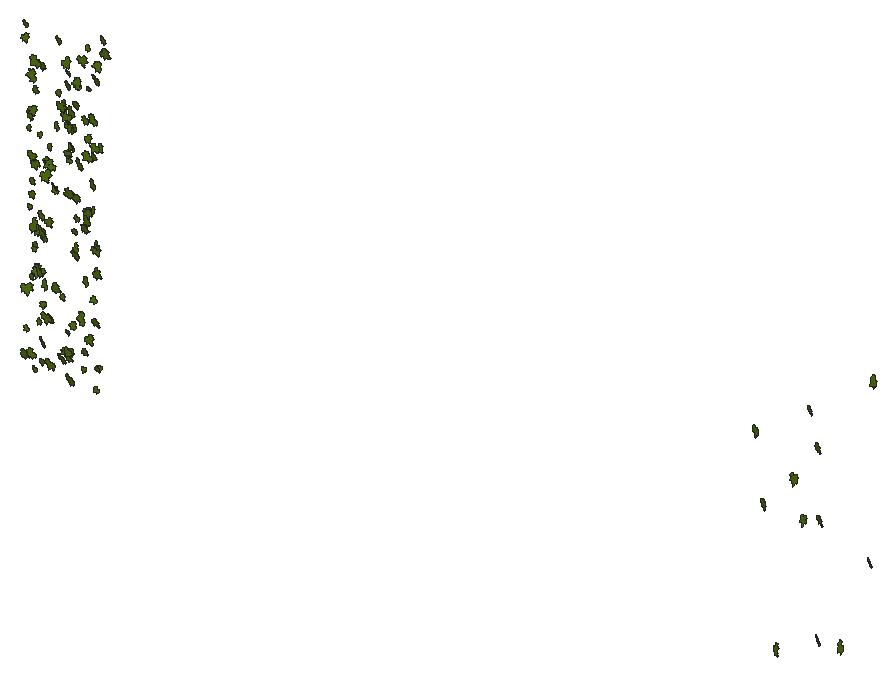
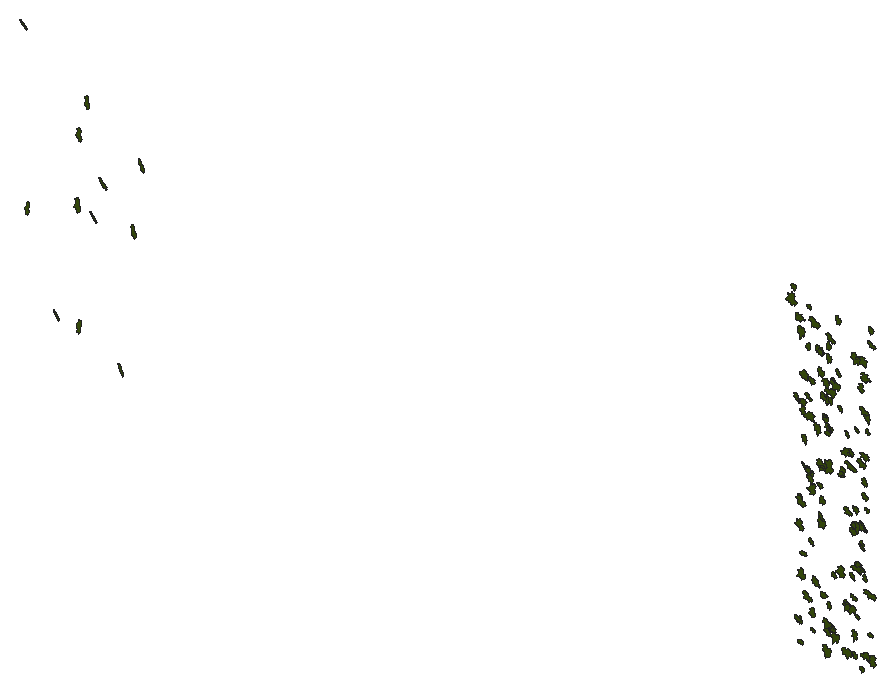
# SketchUp Ruby script. Lengths in inches.
U = 1.inch
M = Sketchup.active_model
def pt(a) = Geom::Point3d.new(a.map { |v| v * U })
def face(e, loops, mat)
  f = e.add_face(loops[0].map { |a| pt(a) })
  loops[1..].each { |l| e.add_face(l.map { |a| pt(a) }).erase! }
  f.material = f.back_material = mat if mat
  f
end
# faces: each face lists its corners as indices into pts; further lists are holes
def faces(e, pts, list, mat = nil) = list.each { |f| face(e, (f[0].is_a?(Array) ? f : [f]).map { |l| l.map { |i| pts[i] } }, mat) }
# xy, xz, yz: faces in a plane at the given z, y or x. An outline is a flat list of corners, or four numbers for a rectangle; further outlines are holes
def ring(l) = l.size == 4 ? [[l[0], l[1]], [l[2], l[1]], [l[2], l[3]], [l[0], l[3]]] : l.each_slice(2).to_a
def flat(e, list, mat, &to3) = list.each { |f| face(e, (f[0].is_a?(Array) ? f : [f]).map { |l| ring(l).map { |u, v| to3.(u, v) } }, mat) }
def xy(e, z, list, mat = nil) = flat(e, list, mat) { |x, y| [x, y, z] }
def xz(e, y, list, mat = nil) = flat(e, list, mat) { |x, z| [x, y, z] }
def yz(e, x, list, mat = nil) = flat(e, list, mat) { |y, z| [x, y, z] }
def lines(e, pts, list) = list.each { |a, b| e.add_line(pt(pts[a]), pt(pts[b])) }
# prism: a flat outline (further loops are holes) pulled along v
def prism(e, loops, v, mat = nil)
  f = face(e, loops, mat); d = Geom::Vector3d.new(v.map { |x| x * U })
  f.pushpull(f.normal.samedirection?(d) ? d.length : -d.length)
end
def box(e, o, s, mat = nil) = prism(e, [[o, [o[0] + s[0], o[1], o[2]], [o[0] + s[0], o[1] + s[1], o[2]], [o[0], o[1] + s[1], o[2]]]], [0, 0, s[2]], mat)
def at(x, y, z, deg = 0) = Geom::Transformation.translation(pt([x, y, z])) * Geom::Transformation.rotation(ORIGIN, Z_AXIS, deg.degrees)
def axes(o, x, y, z) = Geom::Transformation.new([*x, 0, *y, 0, *z, 0, *pt(o).to_a, 1])
def part(name) = M.definitions.add(name)
# library, detail: a bought-in or finely detailed component or shape, given as its bounding box
def library(name, o, s) = part(name).tap { |d| box(d.entities, o, s) }
def detail(e, o, s) = box(e.add_group.entities, o, s)
def put(e, d, t, mat = nil) = e.add_instance(d, t).tap { |i| i.material = mat if mat }
def group(e, t, mat = nil) = e.add_group.tap { |g| g.transformation = t; g.material = mat if mat }.entities
root = M.entities
M.materials.add("[Vegetation Blur 03]").color = [83, 114, 18]
c1 = part("ivy")
xy(c1.entities,0,[[0.782,0,0.786,0,0.787,0.005,0.789,0.009,0.821,0.072,0.875,0.147,1.001,0.272,1.073,0.331,1.137,0.363,1.178,0.379,1.223,0.384,1.272,0.383,1.311,0.374,1.36,0.355,1.399,0.334,1.491,0.285,1.541,0.244,1.583,0.199,1.617,0.15,1.64,0.128,1.662,0.115,1.717,0.105,1.745,0.093,1.784,0.054,1.819,0.057,1.854,0.064,1.882,0.075,1.896,0.074,1.91,0.071,1.937,0.063,1.964,0.053,1.99,0.038,2.016,0.015,2.034,0.002,2.04,0,2.038,0.003,2.036,0.007,2.033,0.038,2.036,0.068,2.045,0.1,2.055,0.116,2.064,0.123,2.077,0.129,2.088,0.129,2.106,0.132,2.118,0.13,2.179,0.132,2.207,0.133,2.225,0.133,2.242,0.138,2.22,0.162,2.207,0.186,2.206,0.213,2.212,0.236,2.228,0.262,2.247,0.274,2.298,0.283,2.355,0.294,2.37,0.296,2.376,0.295,2.377,0.3,2.377,0.303,2.385,0.329,2.411,0.37,2.426,0.392,2.449,0.407,2.511,0.426,2.561,0.444,2.619,0.466,2.589,0.469,2.561,0.476,2.501,0.5,2.449,0.516,2.424,0.523,2.401,0.535,2.377,0.556,2.372,0.568,2.36,0.575,2.268,0.586,2.225,0.592,2.207,0.599,2.194,0.61,2.143,0.65,2.13,0.664,2.122,0.682,2.123,0.7,2.13,0.719,2.148,0.75,2.17,0.781,2.195,0.807,2.221,0.828,2.284,0.874,2.291,0.88,2.288,0.887,2.276,0.9,2.267,0.916,2.265,0.933,2.273,0.967,2.292,1.002,2.313,1.03,2.334,1.054,2.348,1.067,2.358,1.074,2.363,1.076,2.362,1.081,2.35,1.094,2.347,1.11,2.35,1.143,2.359,1.18,2.385,1.254,2.415,1.324,2.448,1.393,2.45,1.4,2.446,1.398,2.44,1.394,2.427,1.383,2.402,1.36,2.376,1.339,2.345,1.324,2.305,1.309,2.282,1.303,2.273,1.306,2.245,1.294,2.212,1.287,2.187,1.291,2.163,1.301,2.142,1.316,2.134,1.327,2.124,1.325,2.09,1.292,2.053,1.259,2.014,1.234,1.973,1.215,1.954,1.21,1.931,1.208,1.909,1.212,1.893,1.22,1.879,1.233,1.872,1.248,1.867,1.281,1.864,1.319,1.821,1.258,1.773,1.197,1.726,1.141,1.698,1.121,1.679,1.116,1.666,1.117,1.647,1.122,1.632,1.129,1.62,1.141,1.617,1.154,1.617,1.219,1.621,1.254,1.623,1.268,1.623,1.281,1.618,1.314,1.606,1.346,1.603,1.375,1.607,1.403,1.603,1.467,1.599,1.499,1.605,1.525,1.614,1.552,1.629,1.577,1.635,1.589,1.629,1.587,1.618,1.582,1.596,1.566,1.581,1.556,1.568,1.552,1.557,1.55,1.545,1.553,1.531,1.562,1.522,1.572,1.504,1.591,1.486,1.611,1.474,1.631,1.457,1.666,1.455,1.684,1.457,1.698,1.452,1.715,1.444,1.728,1.424,1.754,1.419,1.772,1.423,1.786,1.434,1.819,1.444,1.848,1.446,1.855,1.44,1.861,1.43,1.867,1.386,1.904,1.349,1.948,1.326,1.973,1.31,1.995,1.288,2.048,1.284,2.153,1.287,2.254,1.284,2.255,1.282,2.253,1.278,2.247,1.274,2.237,1.266,2.216,1.226,2.125,1.208,2.076,1.184,2.033,1.155,1.984,1.135,1.942,1.111,1.899,1.083,1.861,1.053,1.85,1.059,1.83,1.061,1.809,1.056,1.79,1.049,1.767,1.04,1.749,1.018,1.733,0.994,1.726,0.942,1.734,0.95,1.6875,0.944,1.645,0.932,1.608,0.911,1.585,0.881,1.58,0.854,1.582,0.828,1.588,0.785,1.618,0.773,1.625,0.775,1.614,0.779,1.598,0.796,1.502,0.818,1.402,0.861,1.283,0.882,1.224,0.894,1.174,0.892,1.148,0.886,1.123,0.881,1.107,0.872,1.099,0.849,1.094,0.818,1.092,0.789,1.098,0.762,1.107,0.753,1.113,0.721,1.139,0.698,1.163,0.678,1.194,0.665,1.224,0.628,1.28,0.612,1.312,0.606,1.327,0.606,1.314,0.599,1.282,0.594,1.267,0.581,1.256,0.544,1.245,0.512,1.244,0.473,1.249,0.444,1.256,0.382,1.288,0.339,1.306,0.324,1.316,0.317,1.324,0.309,1.326,0.27,1.314,0.227,1.313,0.185,1.3125,0.152,1.317,0.122,1.328,0.092,1.345,0.073,1.353,0.079,1.338,0.092,1.308,0.117,1.249,0.13,1.215,0.139,1.164,0.147,1.148,0.157,1.136,0.163,1.122,0.174,1.086,0.177,1.067,0.182,1.054,0.186,1.043,0.191,1.038,0.211,1.028,0.237,1.005,0.25,0.974,0.253,0.96,0.25,0.944,0.242,0.914,0.243,0.906,0.249,0.902,0.26,0.894,0.289,0.88,0.307,0.873,0.322,0.862,0.364,0.799,0.403,0.738,0.431,0.709,0.439,0.691,0.441,0.678,0.4375,0.66,0.428,0.645,0.394,0.623,0.303,0.594,0.255,0.581,0.214,0.577,0.179,0.573,0.173,0.568,0.175,0.561,0.167,0.55,0.141,0.523,0.113,0.503,0.077,0.49,0.045,0.486,0.026,0.485,0.019,0.486,0.011,0.483,0,0.471,0.014,0.467,0.044,0.455,0.058,0.447,0.07,0.438,0.097,0.411,0.125,0.394,0.158,0.377,0.174,0.366,0.182,0.359,0.185,0.361,0.242,0.331,0.253,0.316,0.258,0.303,0.262,0.283,0.274,0.278,0.308,0.274,0.341,0.252,0.366,0.226,0.366,0.222,0.37,0.22,0.38,0.221,0.395,0.221,0.425,0.216,0.45,0.207,0.465,0.192,0.473,0.178,0.484,0.15,0.489,0.116,0.483,0.089,0.468,0.058,0.45,0.035,0.435,0.018,0.429,0.011,0.434,0.012,0.438,0.014,0.469,0.019,0.542,0.016,0.581,0.015,0.612,0.027,0.68,0.055,0.696,0.057,0.712,0.052,0.73,0.045,0.741,0.036,0.766,0.014]])
put(root,c1,axes([21.23,173.2,141.55],[0.34233,0.0367,0.25351],[0.30852,-0.16299,-0.27378],[-0.04025,-0.93715,0.05755]),"[Vegetation Blur 03]")
put(root,c1,axes([21.29,173.2,102.73],[0.10484,-0.11239,0.45286],[0.55605,-0.06423,-0.08825],[-0.04094,-1.16025,-0.03898]),"[Vegetation Blur 03]")
put(root,c1,axes([21.54,173.2,143.62],[0.38177,-0.16884,0.00908],[0.01686,0.05275,-0.31784],[-0.08106,-0.78418,-0.02334]),"[Vegetation Blur 03]")
put(root,c1,axes([22.01,173.2,106.74],[0.21979,-0.07452,-0.15702],[-0.1954,-0.04663,-0.1787],[-0.01213,-0.59927,0.03343]),"[Vegetation Blur 03]")
put(root,c1,axes([21.13,173.2,111.34],[0.58242,0.07305,0.2372],[0.29248,-0.20649,-0.46835],[-0.01349,-1.32342,0.08617]),"[Vegetation Blur 03]")
put(root,c1,axes([22.25,173.2,133.14],[0.45147,-0.25025,-0.22719],[-0.26949,0.14362,-0.38159],[-0.1402,-1.08195,0.00189]),"[Vegetation Blur 03]")
put(root,c1,axes([22.05,173.2,130.78],[0.19571,-0.04059,0.18321],[0.21938,-0.10557,-0.15978],[-0.05153,-0.6037,0.01562]),"[Vegetation Blur 03]")
put(root,c1,axes([22.14,173.2,121.49],[0.2893,-0.06946,0.05279],[0.06075,-0.07196,-0.23668],[-0.04039,-0.60575,0.02206]),"[Vegetation Blur 03]")
put(root,c1,axes([22.56,173.2,104.21],[0.3982,-0.07833,-0.27853],[-0.34327,-0.06231,-0.32413],[-0.0091,-1.07738,0.039]),"[Vegetation Blur 03]")
put(root,c1,axes([23.17,173.2,138.125],[0.18243,-0.13935,-0.48722],[-0.59996,0.02639,-0.15082],[-0.03212,-1.28429,0.04976]),"[Vegetation Blur 03]")
put(root,c1,axes([22.41,173.2,112.84],[0.19414,-0.08015,0.20136],[0.24242,-0.09451,-0.1616],[-0.0602,-0.6391,-0.00136]),"[Vegetation Blur 03]")
put(root,c1,axes([22.27,173.2,128.1],[0.54066,-0.11979,-0.01485],[-0.02304,-0.09186,-0.44216],[-0.05647,-1.10941,0.03821]),"[Vegetation Blur 03]")
put(root,c1,axes([22.25,173.2,122.84],[0.30004,-0.03578,0.23182],[0.28092,-0.09842,-0.24458],[-0.04545,-0.84451,0.01868]),"[Vegetation Blur 03]")
put(root,c1,axes([22.36,173.2,124.4375],[0.23733,-0.08095,0.26556],[0.32364,-0.07275,-0.19614],[-0.05179,-0.82556,-0.00876]),"[Vegetation Blur 03]")
put(root,c1,axes([22.15,173.2,133.21],[0.44354,0.00148,0.25414],[0.30752,-0.17731,-0.35733],[-0.04893,-1.101,0.05789]),"[Vegetation Blur 03]")
put(root,c1,axes([22.98,173.2,139.99],[0.532,-0.08529,-0.32199],[-0.3962,-0.04622,-0.4341],[-0.01987,-1.36215,0.03489]),"[Vegetation Blur 03]")
put(root,c1,axes([22.33,173.2,118.68],[0.16553,0.17765,0.51158],[0.60894,-0.40708,-0.109],[-0.17196,-1.2705,0.10646]),"[Vegetation Blur 03]")
put(root,c1,axes([22.85,173.2,102.07],[0.31854,-0.11206,-0.01065],[-0.01233,0.01101,-0.26373],[-0.05462,-0.65595,-0.00261]),"[Vegetation Blur 03]")
put(root,c1,axes([22.77,173.2,116.93],[0.24085,-0.07286,0.19486],[0.23769,-0.04913,-0.19858],[-0.04198,-0.69616,-0.00638]),"[Vegetation Blur 03]")
put(root,c1,axes([23.5,173.2,119.6875],[0.31165,-0.23246,-0.38206],[-0.4746,0.04633,-0.26229],[-0.08166,-1.15634,0.0663]),"[Vegetation Blur 03]")
put(root,c1,axes([22.75,173.2,116.47],[0.2517,0.01272,0.24338],[0.28699,-0.2291,-0.19581],[-0.08127,-0.76965,0.06231]),"[Vegetation Blur 03]")
put(root,c1,axes([22.54,173.2,126.8],[0.46612,-0.06322,0.21313],[0.25778,-0.10592,-0.38046],[-0.05188,-1.09436,0.02451]),"[Vegetation Blur 03]")
put(root,c1,axes([22.89,173.2,135.48],[0.11949,-0.05949,0.35767],[0.43416,-0.12523,-0.09989],[-0.06637,-0.92633,-0.00946]),"[Vegetation Blur 03]")
put(root,c1,axes([23.31,173.2,114.71],[0.56265,-0.26157,-0.25412],[-0.30853,0.09554,-0.47049],[-0.13384,-1.31983,0.01631]),"[Vegetation Blur 03]")
put(root,c1,axes([22.98,173.2,114.27],[0.61939,0.05734,-0.0417],[-0.04546,-0.22498,-0.49845],[0.03634,-1.25897,0.08717]),"[Vegetation Blur 03]")
put(root,c1,axes([23.125,173.2,113.87],[0.12985,0.03067,0.35023],[0.42444,-0.14892,-0.10276],[-0.06505,-0.91052,0.02861]),"[Vegetation Blur 03]")
put(root,c1,axes([23.6,173.2,108.16],[0.30014,-0.14068,-0.03498],[-0.05049,-0.06238,-0.24906],[-0.06295,-0.62077,0.03295]),"[Vegetation Blur 03]")
put(root,c1,axes([23.54,173.2,130.61],[0.25172,-0.04798,0.1294],[0.15152,-0.12662,-0.20371],[-0.0522,-0.59895,0.0327]),"[Vegetation Blur 03]")
put(root,c1,axes([23.64,173.2,119.53],[0.559,-0.25408,-0.226],[-0.26774,0.14716,-0.46713],[-0.14227,-1.27524,-0.00888]),"[Vegetation Blur 03]")
put(root,c1,axes([23.82,173.2,121.35],[0.41365,-0.19736,-0.16762],[-0.20533,0.04633,-0.34609],[-0.09602,-0.94924,0.01796]),"[Vegetation Blur 03]")
put(root,c1,axes([23.34,173.2,139.49],[0.6079,-0.24736,0.08777],[0.11732,0.08596,-0.50313],[-0.11068,-1.26744,-0.05125]),"[Vegetation Blur 03]")
put(root,c1,axes([23.77,173.2,103.27],[0.34382,-0.15266,0.07768],[0.0934,-0.03785,-0.28706],[-0.07642,-0.73315,-0.00136]),"[Vegetation Blur 03]")
put(root,c1,axes([23.8,173.2,106.05],[0.51362,-0.33546,-0.11294],[-0.11227,0.20752,-0.43703],[-0.18199,-1.07476,-0.04914]),"[Vegetation Blur 03]")
put(root,c1,axes([23.84,173.2,110.22],[0.36114,-0.04689,0.10699],[0.12628,-0.12494,-0.29255],[-0.0419,-0.78067,0.04039]),"[Vegetation Blur 03]")
put(root,c1,axes([23.99,173.2,118.66],[0.10493,-0.03643,0.24088],[0.29195,-0.08918,-0.08683],[-0.04677,-0.63839,-0.00162]),"[Vegetation Blur 03]")
put(root,c1,axes([23.96,173.2,118.42],[0.40755,-0.11351,-0.00014],[0.00098,0.01751,-0.33557],[-0.05515,-0.83847,-0.00699]),"[Vegetation Blur 03]")
put(root,c1,axes([24.57,173.2,113.2],[0.33509,-0.2609,-0.26753],[-0.3303,0.08476,-0.28857],[-0.12012,-0.96089,0.04719]),"[Vegetation Blur 03]")
put(root,c1,axes([24.21,173.2,127.48],[0.21376,-0.00368,0.2636],[0.3197,-0.11113,-0.17293],[-0.04601,-0.78924,0.02312]),"[Vegetation Blur 03]")
put(root,c1,axes([23.95,173.2,109.03],[0.66487,-0.12258,0.05657],[0.06821,-0.03171,-0.54475],[-0.06083,-1.37523,0.00752]),"[Vegetation Blur 03]")
put(root,c1,axes([23.78,173.2,125.74],[0.49312,0.07516,0.37451],[0.45503,-0.28887,-0.38996],[-0.06962,-1.3557,0.10386]),"[Vegetation Blur 03]")
put(root,c1,axes([24.4,173.2,120.2],[0.35229,-0.00554,0.29733],[0.36145,-0.12544,-0.28562],[-0.04568,-1.0353,0.03302]),"[Vegetation Blur 03]")
put(root,c1,axes([25.33,173.2,128.11],[0.3559,-0.06669,-0.38571],[-0.47242,-0.14005,-0.28653],[0.03508,-1.20938,0.05445]),"[Vegetation Blur 03]")
put(root,c1,axes([24.67,173.2,103.72],[0.62299,-0.15418,-0.12642],[-0.15294,0.05244,-0.51207],[-0.07884,-1.31998,-0.00558]),"[Vegetation Blur 03]")
put(root,c1,axes([24.82,173.2,129.45],[0.20111,-0.0492,0.23305],[0.27447,-0.17313,-0.16352],[-0.08231,-0.69755,0.02415]),"[Vegetation Blur 03]")
put(root,c1,axes([24.75,173.2,109.0625],[0.49941,-0.26714,0.04177],[0.06827,0.12648,-0.4165],[-0.1217,-1.02529,-0.06226]),"[Vegetation Blur 03]")
put(root,c1,axes([26.03,173.2,124.98],[0.19807,-0.04882,-0.25327],[-0.31096,-0.06252,-0.16009],[0.01294,-0.755,0.02963]),"[Vegetation Blur 03]")
put(root,c1,axes([25.4,173.2,125.22],[0.42582,-0.25778,-0.01572],[0.00049,0.14225,-0.35818],[-0.12674,-0.86554,-0.05419]),"[Vegetation Blur 03]")
put(root,c1,axes([26.12,173.2,132.92],[0.29115,-0.21346,-0.2217],[-0.27097,0.0878,-0.25032],[-0.10549,-0.81469,0.03111]),"[Vegetation Blur 03]")
put(root,c1,axes([25.37,173.2,112.21],[0.18573,-0.07263,0.44986],[0.55141,-0.04477,-0.15278],[-0.03192,-1.19609,-0.0216]),"[Vegetation Blur 03]")
put(root,c1,axes([25.96,173.2,143.22],[0.42985,-0.21428,0.06487],[0.08397,0.02008,-0.36019],[-0.10055,-0.89931,-0.0235]),"[Vegetation Blur 03]")
put(root,c1,axes([25.98,173.2,136.5],[0.26598,-0.07146,0.22657],[0.27016,-0.13937,-0.21816],[-0.07275,-0.7788,0.01825]),"[Vegetation Blur 03]")
put(root,c1,axes([26.15,173.2,104.75],[0.57489,-0.26657,0.03866],[0.06843,0.18847,-0.47339],[-0.11976,-1.17196,-0.08492]),"[Vegetation Blur 03]")
put(root,c1,axes([25.97,173.2,135.15],[0.58643,-0.10608,0.2337],[0.28408,-0.0778,-0.48036],[-0.06289,-1.34069,0.00938]),"[Vegetation Blur 03]")
put(root,c1,axes([26.53,173.2,111.82],[0.22624,-0.03067,0.2044],[0.24637,-0.10398,-0.18409],[-0.04741,-0.6867,0.01875]),"[Vegetation Blur 03]")
put(root,c1,axes([27.13,173.2,105.77],[0.29889,-0.0519,-0.2268],[-0.27904,-0.05258,-0.24304],[-0.001,-0.83818,0.02929]),"[Vegetation Blur 03]")
put(root,c1,axes([26.71,173.2,135.43],[0.18943,-0.02258,0.18927],[0.22327,-0.15119,-0.15168],[-0.06367,-0.59736,0.03124]),"[Vegetation Blur 03]")
put(root,c1,axes([26.93,173.2,134.5625],[0.53942,-0.03341,-0.15907],[-0.19556,-0.07489,-0.43924],[-0.00287,-1.17788,0.03244]),"[Vegetation Blur 03]")
put(root,c1,axes([26.66,173.2,140.22],[0.34036,0.06769,0.40355],[0.48921,-0.24292,-0.26842],[-0.07909,-1.21115,0.07639]),"[Vegetation Blur 03]")
put(root,c1,axes([27.16,173.2,105.97],[0.51001,-0.14732,-0.08686],[-0.10909,-0.02593,-0.41973],[-0.06746,-1.07179,0.02209]),"[Vegetation Blur 03]")
put(root,c1,axes([27.32,173.2,129.21],[0.05918,0.07636,0.27369],[0.32495,-0.20144,-0.03796],[-0.0908,-0.67116,0.04253]),"[Vegetation Blur 03]")
put(root,c1,axes([27.03,173.2,129.69],[0.45211,-0.0957,0.11404],[0.13937,-0.02195,-0.37092],[-0.04759,-0.97354,-0.00285]),"[Vegetation Blur 03]")
put(root,c1,axes([27.25,173.2,107.97],[0.28812,-0.17967,0.12477],[0.15963,0.01216,-0.24278],[-0.07425,-0.67108,-0.0378]),"[Vegetation Blur 03]")
put(root,c1,axes([27.26,173.2,138.25],[0.44121,-0.22953,-0.01023],[-0.00431,0.06987,-0.3705],[-0.11216,-0.9056,-0.026]),"[Vegetation Blur 03]")
put(root,c1,axes([27.75,173.2,129.24],[0.24945,-0.08617,-0.15972],[-0.19859,-0.02674,-0.20432],[-0.02483,-0.6519,0.02949]),"[Vegetation Blur 03]")
put(root,c1,axes([27.27,173.2,139.5625],[0.34754,-0.2147,0.09746],[0.13272,0.06991,-0.29103],[-0.08677,-0.75297,-0.05481]),"[Vegetation Blur 03]")
put(root,c1,axes([27.15,173.2,133.24],[0.58629,-0.17522,0.04019],[0.04988,0.00183,-0.48347],[-0.08478,-1.21072,-0.00655]),"[Vegetation Blur 03]")
put(root,c1,axes([27.08,173.2,124.28],[0.20202,-0.16973,0.51163],[0.63222,0.07532,-0.16235],[0.00985,-1.35325,-0.07321]),"[Vegetation Blur 03]")
put(root,c1,axes([27.39,173.2,104.5],[0.13655,-0.05783,0.35944],[0.43753,-0.10617,-0.1134],[-0.05764,-0.9429,-0.00928]),"[Vegetation Blur 03]")
put(root,c1,axes([27.17,173.2,105.74],[0.52125,-0.12471,0.19571],[0.23821,-0.0569,-0.42827],[-0.06661,-1.17932,-0.00003]),"[Vegetation Blur 03]")
put(root,c1,axes([27.875,173.2,130.86],[0.28246,-0.12607,-0.06429],[-0.08477,-0.04633,-0.23378],[-0.05266,-0.60166,0.03147]),"[Vegetation Blur 03]")
put(root,c1,axes([27.27,173.2,102.72],[0.66178,-0.29714,0.00728],[0.02239,0.12543,-0.55031],[-0.14293,-1.35615,-0.0525]),"[Vegetation Blur 03]")
put(root,c1,axes([27.83,173.2,135.5],[0.50423,-0.25138,-0.23976],[-0.28758,0.12452,-0.42338],[-0.1361,-1.1944,0.00632]),"[Vegetation Blur 03]")
put(root,c1,axes([27.74,173.2,133.44],[0.499,-0.30069,-0.16614],[-0.19194,0.14146,-0.42426],[-0.16109,-1.09995,-0.00914]),"[Vegetation Blur 03]")
put(root,c1,axes([27.78,173.2,131.02],[0.4623,-0.23108,-0.11744],[-0.13279,0.12742,-0.38762],[-0.12523,-0.98816,-0.02252]),"[Vegetation Blur 03]")
put(root,c1,axes([28.76,173.2,109.41],[0.05855,-0.11186,-0.32035],[-0.39567,-0.06136,-0.0448],[0.02177,-0.81436,0.04738]),"[Vegetation Blur 03]")
put(root,c1,axes([27.99,173.2,132.92],[0.26922,-0.1042,0.25304],[0.30661,-0.09593,-0.2235],[-0.06845,-0.83952,-0.00587]),"[Vegetation Blur 03]")
put(root,c1,axes([28.08,173.2,120.4],[0.28875,-0.1223,0.18363],[0.229,0.01809,-0.23796],[-0.04139,-0.75306,-0.03554]),"[Vegetation Blur 03]")
put(root,c1,axes([27.86,173.2,124.96],[0.63148,-0.16792,0.0994],[0.12538,0.04433,-0.51879],[-0.07597,-1.32267,-0.03001]),"[Vegetation Blur 03]")
put(root,c1,axes([27.98,173.2,117.86],[0.52924,-0.21641,0.13482],[0.17446,0.07604,-0.43695],[-0.08896,-1.13835,-0.05482]),"[Vegetation Blur 03]")
put(root,c1,axes([28.29,173.2,118.02],[0.07963,0.08394,0.36792],[0.43963,-0.2386,-0.05481],[-0.10777,-0.91131,0.04824]),"[Vegetation Blur 03]")
put(root,c1,axes([28.84,173.2,138.93],[0.3287,-0.1611,-0.24597],[-0.30329,0.03864,-0.27395],[-0.07054,-0.91688,0.03167]),"[Vegetation Blur 03]")
put(root,c1,axes([28.14,173.2,135.98],[0.42324,-0.15513,0.17492],[0.21736,0.00516,-0.3496],[-0.06611,-0.97622,-0.02964]),"[Vegetation Blur 03]")
put(root,c1,axes([29.29,173.2,139.27],[0.20332,-0.17652,-0.4378],[-0.54125,0.03497,-0.16965],[-0.04646,-1.17997,0.06046]),"[Vegetation Blur 03]")
put(root,c1,axes([28.56,173.2,122.42],[0.35274,-0.11868,-0.02991],[-0.03922,-0.02703,-0.29129],[-0.05595,-0.72928,0.01566]),"[Vegetation Blur 03]")
put(root,c1,axes([28.81,173.2,129.5],[0.58606,-0.32249,-0.17371],[-0.19607,0.18401,-0.49434],[-0.17725,-1.2698,-0.02752]),"[Vegetation Blur 03]")
put(root,c1,axes([29.73,173.2,111.02],[0.29249,-0.26424,-0.46367],[-0.56799,0.1604,-0.25303],[-0.12902,-1.30512,0.06278]),"[Vegetation Blur 03]")
put(root,c1,axes([28.77,173.2,141.69],[0.56787,-0.08069,0.24242],[0.2938,-0.10677,-0.464],[-0.05873,-1.31444,0.02281]),"[Vegetation Blur 03]")
put(root,c1,axes([29.52,173.2,104.3],[0.28663,-0.07213,0.05383],[0.05877,-0.11436,-0.23255],[-0.04609,-0.59433,0.03821]),"[Vegetation Blur 03]")
put(root,c1,axes([30.18,173.2,115.48],[0.25494,-0.21897,-0.29058],[-0.35433,0.12452,-0.22182],[-0.11199,-0.89248,0.04035]),"[Vegetation Blur 03]")
put(root,c1,axes([29.42,173.2,106.08],[0.21568,-0.13397,0.30172],[0.37321,-0.01782,-0.17894],[-0.04036,-0.88058,-0.04228]),"[Vegetation Blur 03]")
put(root,c1,axes([29.6,173.2,134.82],[0.45457,-0.14322,-0.01986],[-0.02603,-0.01905,-0.37516],[-0.06898,-0.93657,0.01067]),"[Vegetation Blur 03]")
put(root,c1,axes([29.47,173.2,120.8],[0.10325,-0.14377,0.42811],[0.52829,-0.03594,-0.08677],[-0.03077,-1.09956,-0.05314]),"[Vegetation Blur 03]")
put(root,c1,axes([30.13,173.2,130.76],[0.44525,-0.05596,-0.30949],[-0.38019,-0.06333,-0.36251],[-0.0007,-1.20185,0.03351]),"[Vegetation Blur 03]")
put(root,c1,axes([30.05,173.2,123.08],[0.46711,-0.27655,-0.25561],[-0.31156,0.09667,-0.39569],[-0.13813,-1.15324,0.02812]),"[Vegetation Blur 03]")
put(root,c1,axes([30.36,173.2,143.71],[0.23115,-0.1069,-0.165],[-0.20647,-0.0259,-0.19002],[-0.03067,-0.63139,0.03573]),"[Vegetation Blur 03]")
put(root,c1,axes([30.73,173.2,123.94],[0.13432,-0.12713,-0.31462],[-0.38869,0.03529,-0.11278],[-0.03669,-0.83931,0.04291]),"[Vegetation Blur 03]")
put(root,c1,axes([29.64,173.2,123.48],[0.52424,-0.12738,0.15619],[0.18843,-0.07357,-0.4307],[-0.07036,-1.14606,0.01029]),"[Vegetation Blur 03]")
put(root,c1,axes([29.85,173.2,132.14],[0.2559,0.03571,0.2999],[0.36108,-0.20047,-0.20147],[-0.07032,-0.89939,0.05682]),"[Vegetation Blur 03]")
put(root,c1,axes([30.16,173.2,138.23],[0.11718,-0.12684,0.22641],[0.28293,-0.00575,-0.09804],[-0.02661,-0.61967,-0.04543]),"[Vegetation Blur 03]")
put(root,c1,axes([29.83,173.2,107.83],[0.38921,-0.01895,0.37093],[0.44943,-0.16908,-0.31546],[-0.06835,-1.21968,0.03797]),"[Vegetation Blur 03]")
put(root,c1,axes([30.86,173.2,135.57],[0.45075,-0.16208,-0.3284],[-0.40131,0.07789,-0.37294],[-0.08406,-1.24093,0.01948]),"[Vegetation Blur 03]")
put(root,c1,axes([30.82,173.2,127.63],[0.43303,-0.27941,-0.22313],[-0.26455,0.14367,-0.37028],[-0.1523,-1.044,0.00876]),"[Vegetation Blur 03]")
put(root,c1,axes([30.7,173.2,123.48],[0.09035,0.0602,0.28294],[0.33236,-0.23291,-0.06289],[-0.10289,-0.69949,0.04529]),"[Vegetation Blur 03]")
put(root,c1,axes([31.15,173.2,113.49],[0.26178,-0.07777,-0.19292],[-0.23918,-0.11506,-0.20887],[0.01,-0.71663,0.05447]),"[Vegetation Blur 03]")
put(root,c1,axes([30.95,173.2,132.04],[0.46854,-0.05722,-0.15501],[-0.19159,-0.07548,-0.38134],[-0.0119,-1.03762,0.03629]),"[Vegetation Blur 03]")
put(root,c1,axes([30.85,173.2,130.125],[0.08947,-0.09548,0.30203],[0.3696,-0.08246,-0.07703],[-0.05008,-0.77914,-0.02886]),"[Vegetation Blur 03]")
put(root,c1,axes([30.86,173.2,140.42],[0.59182,-0.28218,-0.07799],[-0.07654,0.18572,-0.49252],[-0.14859,-1.21956,-0.05695]),"[Vegetation Blur 03]")
put(root,c1,axes([31.4375,173.2,102.625],[0.26116,-0.07939,-0.16142],[-0.20062,-0.0401,-0.21311],[-0.01886,-0.67295,0.03174]),"[Vegetation Blur 03]")
put(root,c1,axes([31.45,173.2,120.29],[0.32555,-0.21056,-0.17248],[-0.21105,0.06347,-0.27751],[-0.10292,-0.79617,0.02349]),"[Vegetation Blur 03]")
put(root,c1,axes([30.76,173.2,110.29],[0.35259,-0.1904,0.31199],[0.38853,0.00444,-0.29204],[-0.06112,-1.07015,-0.05672]),"[Vegetation Blur 03]")
put(root,c1,axes([32.08,173.2,142.18],[0.12519,-0.10736,-0.42184],[-0.51949,-0.03465,-0.1013],[0.00417,-1.09384,0.04461]),"[Vegetation Blur 03]")
put(root,c1,axes([30.66,173.2,119.15],[0.45704,-0.07073,0.34791],[0.42202,-0.13355,-0.37354],[-0.06933,-1.27915,0.01976]),"[Vegetation Blur 03]")
put(root,c1,axes([31.2,173.2,104.6875],[0.21432,-0.13844,0.2244],[0.28013,0.00181,-0.17803],[-0.04065,-0.71738,-0.04375]),"[Vegetation Blur 03]")
put(root,c1,axes([30.98,173.2,115.93],[0.19345,-0.03327,0.47278],[0.57353,-0.16922,-0.15818],[-0.0831,-1.24533,0.00886]),"[Vegetation Blur 03]")
put(root,c1,axes([31.37,173.2,104.98],[0.33883,-0.03876,0.14234],[0.17237,-0.07132,-0.27636],[-0.03256,-0.78094,0.01817]),"[Vegetation Blur 03]")
put(root,c1,axes([31.46,173.2,131.4],[0.18898,0.02634,0.37085],[0.44381,-0.22984,-0.14807],[-0.09838,-0.98629,0.04441]),"[Vegetation Blur 03]")
put(root,c1,axes([32.17,173.2,145.43],[0.36865,-0.17556,-0.1237],[-0.14943,0.05438,-0.30876],[-0.08901,-0.81841,0.00602]),"[Vegetation Blur 03]")
put(root,c1,axes([31.91,173.2,143.01],[0.28018,-0.09633,0.48866],[0.59963,-0.03141,-0.22997],[-0.03369,-1.35996,-0.0293]),"[Vegetation Blur 03]")
put(root,c1,axes([120.07,173.7,128.88],[0.58162,-0.37165,0.13863],[0.15197,-0.16988,-0.49633],[-0.1959,-1.23523,0.02655]),"[Vegetation Blur 03]")
put(root,c1,axes([121.13,173.7,120.18],[0.48124,-0.36893,0.30519],[0.35516,-0.24188,-0.41903],[-0.21409,-1.23057,-0.00913]),"[Vegetation Blur 03]")
put(root,c1,axes([122.83,173.7,102.63],[0.29467,-0.10714,0.44848],[0.50944,-0.44068,-0.23951],[-0.21249,-1.20507,0.04772]),"[Vegetation Blur 03]")
put(root,c1,axes([125.21,173.7,124.85],[0.61028,-0.27277,0.17175],[0.18054,-0.30337,-0.50308],[-0.17106,-1.2933,0.08178]),"[Vegetation Blur 03]")
put(root,c1,axes([126.6,173.7,120.21],[0.50493,-0.24622,0.19162],[0.19585,-0.34808,-0.41408],[-0.17632,-1.09173,0.08881]),"[Vegetation Blur 03]")
put(root,c1,axes([127.46,173.7,133.63],[0.38011,-0.35457,0.334],[0.40396,-0.18413,-0.33696],[-0.18436,-1.13452,-0.04969]),"[Vegetation Blur 03]")
put(root,c1,axes([128.53,173.7,129.17],[0.29678,-0.27186,0.42657],[0.50911,-0.26247,-0.26224],[-0.17731,-1.20867,-0.039]),"[Vegetation Blur 03]")
put(root,c1,axes([128.82,173.7,105.62],[0.09448,-0.24372,0.47773],[0.55916,-0.39227,-0.10514],[-0.20978,-1.15536,-0.06508]),"[Vegetation Blur 03]")
put(root,c1,axes([128.68,173.7,120.64],[0.40386,-0.35784,0.38449],[0.46593,-0.19708,-0.35483],[-0.18733,-1.26162,-0.05362]),"[Vegetation Blur 03]")
put(root,c1,axes([131.97,173.7,107.01],[0.55698,-0.45746,-0.14027],[-0.2006,-0.09744,-0.48055],[-0.19678,-1.19551,0.09284]),"[Vegetation Blur 03]")
put(root,c1,axes([135.71,173.7,117.76],[0.23423,-0.31556,0.37462],[0.44905,-0.24958,-0.22008],[-0.18046,-1.03065,-0.06141]),"[Vegetation Blur 03]")
put(root,c1,axes([136.49,173.7,140.81],[0.4979,-0.40473,-0.18477],[-0.2554,-0.09899,-0.42431],[-0.15719,-1.12116,0.10416]),"[Vegetation Blur 03]")
